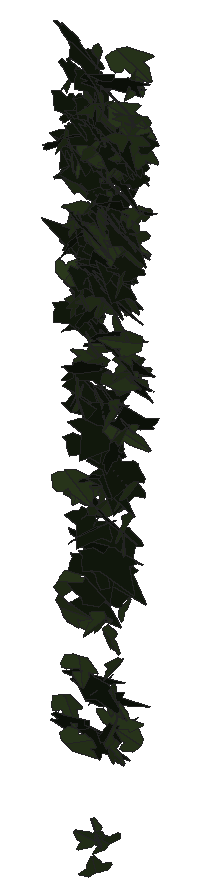
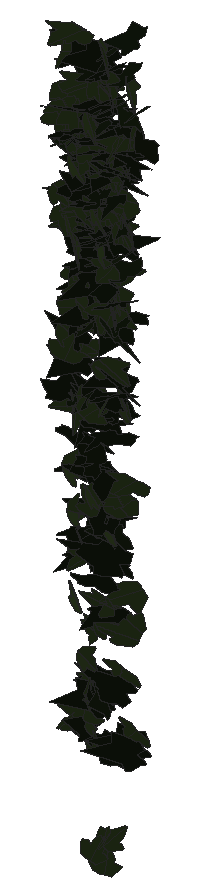
# SketchUp Ruby script. Lengths in millimetres.
U = 1.mm
M = Sketchup.active_model
def pt(a) = Geom::Point3d.new(a.map { |v| v * U })
def face(e, loops, mat)
  f = e.add_face(loops[0].map { |a| pt(a) })
  loops[1..].each { |l| e.add_face(l.map { |a| pt(a) }).erase! }
  f.material = f.back_material = mat if mat
  f
end
# faces: each face lists its corners as indices into pts; further lists are holes
def faces(e, pts, list, mat = nil) = list.each { |f| face(e, (f[0].is_a?(Array) ? f : [f]).map { |l| l.map { |i| pts[i] } }, mat) }
# xy, xz, yz: faces in a plane at the given z, y or x. An outline is a flat list of corners, or four numbers for a rectangle; further outlines are holes
def ring(l) = l.size == 4 ? [[l[0], l[1]], [l[2], l[1]], [l[2], l[3]], [l[0], l[3]]] : l.each_slice(2).to_a
def flat(e, list, mat, &to3) = list.each { |f| face(e, (f[0].is_a?(Array) ? f : [f]).map { |l| ring(l).map { |u, v| to3.(u, v) } }, mat) }
def xy(e, z, list, mat = nil) = flat(e, list, mat) { |x, y| [x, y, z] }
def xz(e, y, list, mat = nil) = flat(e, list, mat) { |x, z| [x, y, z] }
def yz(e, x, list, mat = nil) = flat(e, list, mat) { |y, z| [x, y, z] }
def lines(e, pts, list) = list.each { |a, b| e.add_line(pt(pts[a]), pt(pts[b])) }
# prism: a flat outline (further loops are holes) pulled along v
def prism(e, loops, v, mat = nil)
  f = face(e, loops, mat); d = Geom::Vector3d.new(v.map { |x| x * U })
  f.pushpull(f.normal.samedirection?(d) ? d.length : -d.length)
end
def box(e, o, s, mat = nil) = prism(e, [[o, [o[0] + s[0], o[1], o[2]], [o[0] + s[0], o[1] + s[1], o[2]], [o[0], o[1] + s[1], o[2]]]], [0, 0, s[2]], mat)
def at(x, y, z, deg = 0) = Geom::Transformation.translation(pt([x, y, z])) * Geom::Transformation.rotation(ORIGIN, Z_AXIS, deg.degrees)
def axes(o, x, y, z) = Geom::Transformation.new([*x, 0, *y, 0, *z, 0, *pt(o).to_a, 1])
def part(name) = M.definitions.add(name)
# library, detail: a bought-in or finely detailed component or shape, given as its bounding box
def library(name, o, s) = part(name).tap { |d| box(d.entities, o, s) }
def detail(e, o, s) = box(e.add_group.entities, o, s)
def put(e, d, t, mat = nil) = e.add_instance(d, t).tap { |i| i.material = mat if mat }
def group(e, t, mat = nil) = e.add_group.tap { |g| g.transformation = t; g.material = mat if mat }.entities
root = M.entities
M.materials.add("efeu1").color = [18, 25, 13]
M.materials.add("efeu2").color = [43, 57, 29]
c1 = part("ivyleaf_10")
p = [[0,12.8,-0.8],[-1.5,51.3,-10.9],[-4.9,51,-11.6],[-13.6,26.5,-7.3],[-13.2,15.9,-4.6],[-21.1,19.3,-7.2],
  [-29.5,16.3,-8.3],[-29.2,8.3,-6.2],[-19.7,-9.8,0.5],[-7.6,-13,4],[1,-12.2,5.8],[-0.4,51.1,-11.1],
  [-1.5,51.1,-10.9],[1,-12.4,5.9],[16.9,-12.4,3.5],[35.1,9.1,-5.1],[35,12.9,-6.1],[20.5,16.4,-4.9],
  [15.8,15,-3.8],[15.3,27.6,-7.1],[12.8,31.3,-7.8]]
faces(c1.entities,p,[[0,1,2,3,4,5,6,7,8,9,10],[11,12,0,13,14,15,16,17,18,19,20]],"efeu2")
c2 = part("ivyleaf_9")
p = [[39.1,54.8,31.7],[34.5,51.8,30.2],[-5.3,25.2,17.3],[-17.9,28.3,20.9],[-21.6,21.7,17],[-20.2,4.3,5.3],
  [-22.9,-0.3,2.5],[-17.1,-4,-0.6],[-2,-2.1,-1.2],[-0.7,-15.4,-10.1],[16.6,-22.3,-16.7],[21.1,-15.1,-12.5],
  [32.7,-10.7,-11],[46.1,-1.8,-6.6],[30.8,11.2,3.8]]
faces(c2.entities,p,[[0,1,2,3,4,5,6,7,8,9,10,11,12,13,14]],"efeu1")
put(root,c1,axes([2306.4,958.9,65.1],[-0.49268,-0.36082,-0.57278],[-0.62271,-0.47016,0.44405],[-1.12791,0.41718,0.00504]))
put(root,c1,axes([2262.1,935.2,1434.6],[-0.09896,-0.49853,-0.72888],[0.15767,0.72417,-0.50121],[1.67323,-0.09772,0.00412]))
put(root,c1,axes([2339.9,936.6,1299.7],[-0.34814,0.53797,0.53709],[-0.43479,0.48799,-0.56659],[-1.37991,-0.28948,0.04302]))
put(root,c2,axes([2364.3,933.3,858.2],[0.11458,-0.04516,-0.89711],[-1.05775,0.70448,-0.07276],[1.34302,0.55869,0.01923]))
put(root,c1,axes([2315,956.2,10],[-0.58701,-0.59557,-0.27554],[-0.24044,-0.24487,0.6707],[-1.22555,0.3333,0.00039]))
put(root,c1,axes([2391.6,960.3,1066.8],[-0.12621,-0.04578,-0.84309],[-1.31279,-0.48478,0.08058],[-0.92673,0.69296,0.00067]))
put(root,c2,axes([2326.7,937,1518.4],[0.06754,0.0188,-0.84588],[-1.42002,0.39992,-0.02242],[0.75932,0.74622,0.03332]))
put(root,c2,axes([2369.8,956.2,826.1],[-1.39765,-0.25317,-0.39205],[0.68805,0.15365,-0.7764],[0.56169,-0.81817,-0.02449]))
put(root,c1,axes([2370.8,960.3,1191],[0.433,-0.53815,0.4661],[0.34565,-0.42926,-0.58427],[1.31013,0.29111,0.0001]))
put(root,c2,axes([2307.6,962.7,686.4],[-0.82925,-0.62066,0.17912],[-0.18279,-0.15142,-0.75829],[1.21579,-0.4461,0.00817]))
put(root,c1,axes([2382.1,949.2,898.1],[0.07989,-0.81763,-0.16606],[-0.0415,0.16514,-0.81861],[1.58735,0.04547,-0.01304]))
put(root,c1,axes([2265.1,945.8,765],[1.24363,0.38111,0.45401],[0.69616,0.27249,-0.75519],[-0.88774,0.74757,0.04381]))
put(root,c1,axes([2339.9,961,258.8],[-0.14365,0.06886,-0.76785],[0.7937,-0.64524,-0.09886],[-1.23402,-0.42303,0.02579]))
put(root,c1,axes([2329.4,951.7,1511],[-0.57099,-0.84663,0.00578],[-0.0035,-0.00548,-0.89821],[1.61134,-0.30002,0.0001]))
put(root,c2,axes([2285.6,960.8,1596.7],[0.20531,-0.82442,0.12259],[0.05769,-0.11965,-0.83133],[1.58524,0.11113,0.01438]))
put(root,c1,axes([2247.9,956.1,496.2],[-0.64764,0.06535,0.7255],[1.33715,-0.18204,0.34593],[0.36614,0.78039,0.01994]))
put(root,c2,axes([2323.5,960.6,1292.1],[0.54514,-0.50862,0.53213],[0.58938,-0.43475,-0.58223],[1.27096,0.41976,0.04176]))
put(root,c2,axes([2312.2,955.2,610.5],[-0.91404,-0.30528,-0.63224],[1.06895,0.29255,-0.56791],[0.80174,-0.7381,0.0364]))
put(root,c1,axes([2342.6,961.6,352.1],[0.12018,-0.03133,0.7733],[1.18762,-0.45689,-0.06946],[0.8713,0.62708,-0.01198]))
put(root,c2,axes([2330.9,963.7,1539.4],[0.31518,-0.57207,0.58879],[0.5868,-0.51334,-0.58548],[1.44802,0.33254,0.1091]))
put(root,c1,axes([2360.7,960.5,1415.5],[-0.03448,-0.74129,0.37323],[0.13613,-0.37332,-0.738],[1.57367,0.01605,0.07202]))
put(root,c2,axes([2367.3,938.8,1578.5],[1.16505,0.56513,0.13133],[0.19397,0.08321,-0.83309],[-1.08706,0.62053,-0.0079]))
put(root,c2,axes([2348,951.5,786.5],[0.66856,-0.64102,-0.32987],[-0.30642,0.28793,-0.73096],[1.3374,0.38641,-0.00257]))
put(root,c1,axes([2324.6,940,1047.8],[-0.13988,-0.08981,-0.73061],[0.88419,0.56387,-0.11605],[1.08668,-0.47036,0.00038]))
put(root,c2,axes([2306.7,936,1092.5],[0.0999,0.44209,0.63564],[0.05692,0.63547,-0.44444],[-1.47248,0.05456,0.02594]))
put(root,c2,axes([2341.4,957.4,1181.5],[1.18471,-0.05553,0.53195],[-1.00217,0.07936,0.62447],[-0.17832,-0.81496,0.02456]))
put(root,c2,axes([2326.7,965.1,869.8],[-1.15879,-0.60672,0.12312],[-0.14494,-0.09798,-0.85941],[1.1693,-0.61342,0.01549]))
put(root,c1,axes([2281.5,956.7,1120.1],[0.17079,-0.89177,0.10539],[0.04625,-0.10347,-0.89616],[1.7084,0.09195,0.01373]))
put(root,c1,axes([2321.6,941.5,1038.5],[-0.23686,0.42105,-0.59435],[-0.50329,0.5357,0.43488],[1.29166,0.28594,0.06046]))
put(root,c1,axes([2388.8,951.2,1469.7],[-1.25192,-0.4557,-0.05778],[0.11272,0.01594,-0.79996],[0.86693,-0.66014,0.02057]))
put(root,c2,axes([2302.3,955.2,373.4],[-0.10895,-0.04436,-0.82621],[1.51762,0.21799,-0.06695],[0.42011,-0.79898,0.0276]))
put(root,c2,axes([2253,935.1,1424.6],[0.91317,0.7112,0.3862],[0.42487,0.31524,-0.85788],[-1.48048,0.52914,-0.00799]))
put(root,c1,axes([2275.1,956.3,403.8],[1.3541,-0.17134,0.27035],[0.50338,-0.05634,-0.7318],[0.34303,0.75903,0.0067]))
put(root,c2,axes([2322.7,956.3,1164],[0.57464,-0.69926,-0.17699],[-0.15447,0.15771,-0.76157],[1.36407,0.31243,-0.01169]))
put(root,c1,axes([2299.9,939.5,1136.5],[-0.23265,0.26561,0.72242],[-0.71916,0.61655,-0.29062],[-1.27621,-0.39585,0.03207]))
put(root,c2,axes([2336.6,953.1,634.5],[-0.43068,-0.50109,-0.65626],[0.68549,0.55241,-0.54598],[1.41407,-0.4204,0.0648]))
put(root,c1,axes([2335,952.3,1238.3],[1.01929,-0.23189,-0.50994],[-0.90114,0.18962,-0.58351],[0.56974,0.71478,-0.01063]))
put(root,c1,axes([2339.1,959,1331.4],[0.71851,-0.68155,0.1673],[0.15577,-0.14592,-0.77912],[1.32652,0.3863,0.00087]))
put(root,c2,axes([2244.5,960,1629.9],[0.95168,-0.69895,0.12172],[0.14261,-0.09605,-0.85939],[1.34272,0.5056,0.00501]))
put(root,c1,axes([2362.5,949.4,982.3],[-0.6751,-0.52179,0.45423],[0.45155,0.38775,0.6307],[-1.23679,0.42639,-0.01768]))
put(root,c1,axes([2313.4,952.9,1319.8],[0.13235,-0.75524,-0.18981],[0.06197,0.19322,-0.75687],[1.48077,0.05942,0.04864]))
put(root,c2,axes([2345.9,949.1,1435.6],[0.71762,-0.51834,-0.57077],[-0.56885,0.48742,-0.64009],[1.35264,0.47998,0.03362]))
put(root,c2,axes([2292.1,952.2,849.8],[-0.01846,-0.53903,-0.59916],[0.27403,0.5884,-0.53169],[1.5092,-0.11343,0.08921]))
put(root,c2,axes([2333.1,937.8,1060.8],[0.99668,0.38051,0.68488],[1.01112,0.43301,-0.6468],[-1.09596,0.74553,0.02611]))
put(root,c2,axes([2349.7,971.7,1166.7],[-0.57073,-0.57735,0.46408],[0.17755,-0.52612,-0.59425],[1.39857,-0.16882,0.26482]))
put(root,c2,axes([2280.7,954.4,1171],[0.70169,-0.62159,-0.33271],[-0.11659,0.34579,-0.71392],[1.33674,0.35645,0.11238]))
put(root,c2,axes([2315.5,965.3,1478.2],[0.40839,-0.77793,0.15754],[0.13852,-0.14323,-0.80637],[1.50426,0.22439,0.03148]))
put(root,c1,axes([2288.3,941.2,928.5],[-0.31168,0.22479,0.89507],[-1.21526,0.62872,-0.27473],[-1.26809,-0.65778,0.04329]))
put(root,c2,axes([2353,962.6,1457.9],[-0.34576,-0.01208,-0.80373],[1.52872,-0.03401,-0.18105],[-0.05808,-0.8233,0.01927]))
put(root,c2,axes([2311.5,944.6,1557.9],[1.04687,0.15062,0.6169],[1.10269,0.21502,-0.56911],[-0.49467,0.79806,0.0369]))
put(root,c1,axes([2262.5,942.1,1161.3],[0.61198,0.28852,-0.63424],[0.36914,0.63384,0.38668],[1.2737,-0.32233,0.19267]))
put(root,c2,axes([2270.5,957.6,1092.7],[-0.39574,-0.59761,-0.51311],[0.39568,0.47022,-0.63191],[1.44591,-0.29224,0.03249]))
put(root,c2,axes([2282.5,960.6,1239],[-0.42881,0.51676,-0.53556],[0.39076,-0.49469,-0.5637],[-1.36143,-0.30475,0.00689]))
put(root,c1,axes([2343.4,955.3,277.1],[0.61445,-0.76799,0.1296],[-0.09504,0.1196,0.83309],[-1.47925,-0.32669,0.00031]))
put(root,c1,axes([2301.7,961,1254.8],[-0.96415,0.31057,-0.50559],[0.66696,-0.37986,-0.58447],[-0.91128,-0.6066,0.10715]))
put(root,c1,axes([2325.3,957.5,1128.6],[-0.93487,-0.65682,0.02553],[-0.02903,-0.02047,-0.82018],[1.25066,-0.49144,0.00004]))
put(root,c2,axes([2313,960.2,1377.1],[1.1269,-0.54134,0.14898],[0.21056,-0.09978,-0.80227],[1.04764,0.60235,0.001]))
put(root,c1,axes([2346.3,974.4,915.6],[0.16756,-0.37842,0.85664],[0.47516,-0.81979,-0.38781],[1.71785,0.26367,0.02371]))
put(root,c2,axes([2326.2,969,1221.5],[-0.31714,-0.761,0.11539],[-0.00562,-0.11743,-0.77872],[1.46487,-0.1652,0.02199]))
put(root,c1,axes([2388.1,968,1027],[-0.28112,-0.68776,0.50868],[-0.17205,-0.50077,-0.70332],[1.61895,-0.17264,0.01359]))
put(root,c1,axes([2310.1,953,1406.5],[1.30656,0.11248,-0.49154],[0.9245,0.07522,0.69565],[0.25744,-0.84098,-0.00352]))
put(root,c2,axes([2253.9,960.4,1560.5],[0.8708,-0.69505,-0.09896],[-0.07819,0.09141,-0.83198],[1.33386,0.45912,0.01584]))
put(root,c2,axes([2296.8,961.3,1220.8],[-0.01863,0.0925,0.81453],[-1.55555,0.06158,-0.01681],[-0.12005,-0.81226,0.09148]))
put(root,c2,axes([2386.3,963.1,1220],[-1.36769,0.06407,0.43761],[-0.83493,0.00266,-0.72081],[-0.10678,-0.84138,0.03104]))
put(root,c2,axes([2301.6,963.8,1553.1],[0.05436,-0.81659,-0.19197],[-0.05508,0.19101,-0.81681],[1.59556,0.03441,-0.02166]))
put(root,c2,axes([2265.1,965.3,1270.2],[1.03589,-0.78141,0.18703],[0.18881,-0.15881,-0.95225],[1.51749,0.55318,-0.00919]))
put(root,c2,axes([2295.4,957.5,1453.8],[-0.08359,-0.58968,-0.56458],[0.38041,0.54042,-0.58],[1.50644,-0.16919,0.11513]))
put(root,c2,axes([2336.4,964.8,1055],[0.67121,-0.73903,0.03827],[0.03313,-0.0341,-0.81887],[1.40801,0.3531,0.00102]))
put(root,c1,axes([2305.9,974,1188.2],[0.12508,-0.35407,-0.79019],[0.23053,-0.78091,0.35999],[-1.63177,-0.13747,-0.00971]))
put(root,c1,axes([2311.3,954.4,1535.7],[1.19509,-0.42437,-0.34252],[-0.26517,0.38019,-0.72647],[1.00346,0.60587,0.21595]))
put(root,c1,axes([2262.8,962.9,905],[0.49836,-0.71309,-0.12686],[0.08368,-0.11899,0.75965],[-1.37592,-0.26552,0.00025]))
put(root,c2,axes([2364.6,961.2,1280.1],[0.40682,-0.72505,-0.31162],[-0.09139,0.3103,-0.75492],[1.49919,0.21566,0.03854]))
put(root,c1,axes([2310.1,974.6,489.3],[-0.0038,-0.30282,0.71041],[0.15738,-0.70641,-0.30089],[1.46131,0.07529,0.03425]))
put(root,c2,axes([2325,963.4,1228],[-0.60239,-0.60485,-0.43687],[0.35425,0.39554,-0.68248],[1.37512,-0.36686,-0.01556]))
put(root,c1,axes([2386.8,963.3,991.4],[-1.05882,-0.48954,0.26481],[-0.37666,-0.17595,-0.74105],[0.99003,-0.59049,0.00127]))
put(root,c2,axes([2242.5,968,1487.7],[0.31044,-0.82332,-0.03787],[-0.00209,0.03838,-0.8393],[1.5686,0.16299,0.00638]))
put(root,c1,axes([2290,966.2,1293.3],[-0.84575,-0.65768,0.26278],[-0.11124,-0.27511,-0.78738],[1.34331,-0.43686,0.10025]))
put(root,c1,axes([2272.3,967.3,1260.1],[-0.22311,-0.743,0.24242],[0.05368,-0.249,-0.74951],[1.48647,-0.10253,0.06345]))
put(root,c1,axes([2375.3,976.8,770.4],[0.29431,-0.56166,0.72735],[0.28271,-0.7126,-0.58185],[1.72598,0.21249,-0.02872]))
put(root,c1,axes([2328.7,971.3,470.7],[-0.28013,0.19766,-0.6896],[0.62361,-0.60772,-0.24413],[-1.21455,-0.35762,0.0337]))
put(root,c2,axes([2384.8,967.8,898.9],[1.04434,0.18542,0.54182],[-0.97085,-0.18278,0.57917],[0.49534,-0.74918,-0.0072]))
put(root,c2,axes([2344.8,969.3,1375.5],[0.68535,-0.7032,0.15678],[0.09391,-0.15079,-0.78967],[1.36798,0.36265,-0.02434]))
put(root,c1,axes([2287.3,969.4,659.7],[0.14512,-0.6073,-0.35431],[0.242,-0.3386,0.60773],[-1.31607,-0.12923,0.07268]))
put(root,c1,axes([2315.1,952.9,1426.2],[-0.50838,-0.54805,-0.55714],[0.55436,0.47655,-0.60842],[1.38021,-0.39327,0.03916]))
put(root,c1,axes([2347.9,960.5,1496.3],[-1.45122,-0.26645,0.11069],[-0.21436,-0.01306,-0.80736],[0.50556,-0.7704,-0.0246]))
put(root,c2,axes([2287.7,958.4,892.9],[-0.23123,0.00874,0.81576],[1.51789,-0.17226,0.12063],[0.32668,0.80657,0.01692]))
put(root,c2,axes([2306.4,964.7,1074.7],[0.98372,-0.65093,-0.05961],[-0.07383,0.04531,-0.83118],[1.24184,0.51833,-0.0022]))
put(root,c2,axes([2306.1,969.4,705.4],[0.88392,-0.54922,0.45596],[0.59049,-0.33458,-0.71905],[1.2235,0.55826,0.01763]))
put(root,c2,axes([2273.4,944.7,1477.6],[0.40889,0.45839,0.65824],[0.02212,0.67959,-0.47705],[-1.52643,0.13264,0.16941]))
put(root,c2,axes([2289.7,946.4,659.7],[-0.21321,0.64599,-0.46863],[-0.14726,0.46221,0.65563],[1.51174,0.13613,-0.00223]))
put(root,c2,axes([2332,956.5,547.9],[-1.5984,-0.05646,0.23177],[0.44037,0.01359,0.84174],[-0.11047,0.87114,0.00189]))
put(root,c1,axes([2364.6,965.7,1225.8],[-1.50236,-0.00174,0.28742],[0.54701,-0.01148,0.78931],[0.00436,0.84001,0.01138]))
put(root,c1,axes([2254.8,949.4,558.9],[-0.42445,-0.224,-0.88221],[1.08422,0.67406,-0.31516],[1.35106,-0.6113,-0.02425]))
put(root,c2,axes([2358.5,973.2,1016.9],[0.33075,-0.22307,0.73051],[0.76608,-0.60996,-0.28202],[1.23545,0.43795,-0.0207]))
put(root,c1,axes([2261.3,961.4,240],[0.90553,0.00884,-0.63596],[1.21014,0.01184,0.47587],[0.02813,-0.79415,0.00002]))
put(root,c2,axes([2237.8,959.7,275],[1.20585,-0.06482,0.47014],[0.88874,-0.05472,-0.63687],[0.1611,0.78706,-0.00556]))
put(root,c1,axes([2358.5,971.1,1400.7],[-0.665,-0.67022,0.29406],[-0.01538,-0.3223,-0.74419],[1.39286,-0.32355,0.13218]))
put(root,c2,axes([2287.5,970.8,1237.1],[0.35103,-0.76454,-0.04074],[-0.0017,0.04169,-0.78642],[1.45713,0.18423,0.0089]))
put(root,c1,axes([2255.7,963.7,1541.9],[0.25173,-0.8257,-0.16833],[0.00152,0.17052,-0.83579],[1.6038,0.12944,0.02721]))
put(root,c2,axes([2345.8,960.1,607.5],[0.17232,-0.55616,-0.63736],[0.11555,0.64362,-0.553],[1.60577,0.01337,0.10819]))
put(root,c1,axes([2341.7,975.5,1088.9],[0.08698,-0.17408,0.78669],[1.22665,-0.46496,-0.14033],[0.92023,0.63623,0.1127]))
put(root,c1,axes([2358.5,960.4,886],[0.65027,0.1764,0.68235],[1.18057,0.2847,-0.38421],[-0.63674,0.70801,-0.01551]))
put(root,c1,axes([2290.1,962.8,1242.4],[-0.84638,0.70787,-0.06223],[-0.07385,0.04911,0.83595],[1.3504,0.44635,0.00671]))
put(root,c2,axes([2296.6,968.3,1497.6],[0.25347,-0.79396,-0.27331],[0.04785,0.28038,-0.80223],[1.59738,0.11759,0.0674]))
put(root,c2,axes([2309.7,964.3,1362.9],[-1.50326,-0.33319,-0.19865],[-0.32068,-0.11122,0.8565],[-0.66499,0.80683,0.03603]))
put(root,c2,axes([2304,964.1,1144.2],[1.57695,-0.34182,0.18948],[0.32103,-0.08788,-0.89616],[0.67096,0.84541,-0.01654]))
put(root,c2,axes([2333.4,964.3,1271.9],[1.35679,-0.30211,0.154],[0.2612,-0.07078,-0.77419],[0.59015,0.7259,-0.01139]))
put(root,c2,axes([2317.4,965.3,1285.5],[0.8223,-0.62245,-0.24071],[-0.13331,0.24287,-0.75377],[1.26312,0.43085,0.07715]))
put(root,c2,axes([2268.2,963.4,368.6],[1.11645,0.32956,-0.39131],[0.61921,0.21914,0.67229],[0.75141,-0.67024,0.0274]))
put(root,c2,axes([2281.3,968.8,253.7],[0.75627,-0.07569,-0.68942],[1.28534,0.22307,0.36477],[0.30043,-0.76383,0.17485]))
put(root,c1,axes([2234.8,971.2,306.5],[1.1218,-0.1697,0.4472],[0.81644,-0.12637,-0.61337],[0.40268,0.72901,-0.00222]))
put(root,c2,axes([2322.8,974.7,1333.3],[-0.06764,-0.79116,-0.10623],[0.03478,0.1055,-0.79184],[1.51884,-0.03765,0.0134]))
put(root,c2,axes([2352,977.4,779.8],[-0.88177,-0.71241,-0.10635],[0.1071,0.09027,-0.84981],[1.36669,-0.46671,-0.00202]))
put(root,c1,axes([2345.1,976.2,417.7],[0.03916,-0.62016,0.37202],[0.00704,-0.37207,-0.62046],[1.37635,0.01955,-0.00741]))
put(root,c1,axes([2259.7,966.6,1273.7],[0.50171,-0.71139,-0.19754],[-0.12229,0.18685,-0.75865],[1.39982,0.27129,0.00452]))
put(root,c2,axes([2300.1,968.1,1459.5],[1.00589,-0.60117,-0.18155],[-0.16444,0.16542,-0.7993],[1.18382,0.53379,0.04324]))
put(root,c2,axes([2286.3,978.6,936.5],[-0.61902,-0.70375,0.01057],[0.00898,-0.01383,-0.77521],[1.33949,-0.32513,0.01008]))
put(root,c2,axes([2327.1,960.8,782.5],[0.48248,0.74846,-0.2114],[-0.13017,-0.20003,-0.79022],[-1.47446,0.26257,0.00059]))
put(root,c1,axes([2270.8,971.3,742.2],[0.82676,0.50582,-0.23347],[-0.31974,-0.16333,-0.66646],[-1.01091,0.46534,0.01985]))
put(root,c2,axes([2310.7,979.6,801.2],[0.84523,-0.13885,-0.6961],[1.25317,-0.22608,0.46519],[-0.50454,-0.79416,-0.01072]))
put(root,c2,axes([2262.2,974.8,1212],[0.36932,-0.73731,-0.05239],[-0.0219,0.05115,-0.76241],[1.40661,0.19438,0.00188]))
put(root,c1,axes([2382.5,982.9,1571.1],[0.07826,0.43246,-0.78849],[-0.23633,-0.77903,-0.43374],[-1.69516,0.12857,0.02407]))
put(root,c1,axes([2267.1,967.1,719.7],[-0.91719,-0.35196,0.41518],[0.6288,0.25151,0.59672],[-0.8232,0.58426,-0.00677]))
put(root,c2,axes([2334.2,971.2,1176.6],[-0.20982,-0.68489,-0.45434],[0.16853,0.44584,-0.69357],[1.55511,-0.14072,0.01386]))
put(root,c2,axes([2335.4,980.8,1467.3],[-0.44173,-0.07874,0.763],[-1.36562,-0.25948,-0.24505],[0.516,-0.75413,0.00465]))
put(root,c2,axes([2277.5,963.2,1071.6],[1.45088,-0.0328,-0.37748],[-0.71328,0.05955,-0.76205],[0.10614,0.84859,0.03888]))
put(root,c1,axes([2315.7,969.4,707.4],[-0.50543,-0.77695,0.23113],[0.2276,0.203,0.81981],[-1.52585,0.28764,0.04573]))
put(root,c1,axes([2320.2,974.2,1284.2],[0.05554,-0.79936,0.0857],[0.01325,-0.0855,-0.79989],[1.53001,0.02976,0.00381]))
put(root,c2,axes([2305.8,982.4,1313.3],[0.53066,-0.66473,0.43253],[0.27978,-0.40722,-0.7206],[1.4832,0.31464,-0.01883]))
put(root,c1,axes([2298.8,971.7,85.9],[-0.31483,0.66989,-0.17543],[0.08139,-0.17014,-0.69001],[-1.31541,-0.17086,-0.0007]))
put(root,c1,axes([2357.3,959.7,1508.8],[0.59548,0.39375,0.66475],[0.59351,0.59181,-0.49733],[-1.34534,0.43537,0.07483]))
put(root,c2,axes([2325.6,959.5,1303.3],[0.83561,0.11727,0.70979],[1.26221,0.25625,-0.45257],[-0.53057,0.7943,0.04121]))
put(root,c1,axes([2382.9,973,1495.4],[-0.93105,-0.66717,0.05283],[0.01668,-0.07182,-0.82582],[1.27362,-0.48678,0.04944]))
put(root,c1,axes([2380.6,978.5,273.4],[-0.02635,0.59627,0.47066],[-0.03985,-0.47086,0.5959],[1.4452,-0.00211,0.02501]))
put(root,c2,axes([2270,960,979],[1.13834,0.33004,0.3442],[0.57795,0.16211,-0.68312],[-0.69977,0.67078,-0.00427]))
put(root,c2,axes([2340.9,957.3,273.6],[0.01261,0.03793,0.80643],[1.04802,0.58952,-0.03225],[-1.12359,0.5503,-0.02103]))
put(root,c1,axes([2334.8,963.3,1132.8],[-0.64965,-0.27715,-0.64569],[0.99194,0.38158,-0.43931],[0.8969,-0.62276,0.01818]))
put(root,c1,axes([2329.6,984.9,351.5],[0.27989,-0.39968,0.69972],[0.77946,-0.57549,-0.4148],[1.3208,0.42432,0.09651]))
put(root,c1,axes([2306.8,971.4,1596.1],[0.59311,-0.76022,-0.18841],[-0.01371,0.19998,-0.81884],[1.49056,0.30434,0.06744]))
put(root,c2,axes([2343.2,981.5,1286.8],[-1.17196,-0.06983,0.43979],[-0.80136,-0.15294,-0.61384],[0.27581,-0.74109,0.08524]))
put(root,c1,axes([2358.6,988.5,696.5],[0.3198,-0.43379,0.74037],[0.44665,-0.70244,-0.46483],[1.57086,0.28804,-0.01856]))
put(root,c2,axes([2241.7,986.7,1192.2],[0.0798,-0.62521,0.47513],[0.36084,-0.45367,-0.6137],[1.45029,0.14728,0.12655]))
put(root,c1,axes([2268.7,980.6,1127],[-0.38995,0.5131,-0.49031],[0.16503,-0.48841,-0.54735],[-1.34058,-0.20937,0.07524]))
put(root,c1,axes([2294.5,980.1,995.5],[-0.75276,-0.42422,0.48369],[-0.60217,-0.36611,-0.57983],[1.06615,-0.50631,0.01401]))
put(root,c1,axes([2359.3,966.6,1250.8],[-0.35512,-0.42334,-0.62517],[1.08916,0.34075,-0.40155],[0.9373,-0.55636,0.22975]))
put(root,c2,axes([2336.7,963.1,1304.6],[-0.2716,-0.17651,0.84402],[1.37977,0.4386,0.2143],[-0.88848,0.73509,0.0748]))
put(root,c1,axes([2243.6,980,1328.1],[-0.57209,0.19641,-0.75857],[1.1472,-0.46117,-0.35826],[-0.95288,-0.67314,0.02411]))
put(root,c2,axes([2275.7,966.5,1334.6],[1.09265,-0.19969,-0.53388],[-0.88868,0.26982,-0.60305],[0.62217,0.73609,0.07622]))
put(root,c1,axes([2365.7,970.2,1140.8],[-1.1792,0.35525,0.16784],[-0.30649,0.05627,-0.71356],[-0.68207,-0.63945,0.03046]))
put(root,c1,axes([2330.5,972.4,1418.6],[1.25793,0.3724,0.21897],[0.31791,0.1488,-0.75726],[-0.75824,0.6802,0.04577]))
put(root,c1,axes([2298.9,977.7,927.6],[-0.50836,0.68467,-0.33979],[0.23525,-0.31651,-0.73493],[-1.43556,-0.29432,-0.00011]))
put(root,c1,axes([2316.9,987.2,50.3],[-0.4587,-0.46735,-0.58776],[-0.39854,-0.55097,0.52397],[-1.37245,0.31619,0.04429]))
put(root,c2,axes([2281.1,988.4,1119.6],[-0.75333,-0.61012,0.23934],[-0.14023,-0.2364,-0.7245],[1.23943,-0.39758,0.0635]))
put(root,c1,axes([2346.4,987.2,663.4],[0.26359,-0.21962,0.72972],[0.89909,-0.55722,-0.25737],[1.13804,0.4911,0.03431]))
put(root,c2,axes([2312.9,971.7,1404.9],[-1.20859,-0.42973,0.35723],[0.61619,0.15782,0.76539],[-0.86687,0.71132,0.046]))
put(root,c1,axes([2375.8,983.7,990.2],[-0.96361,-0.48638,-0.37022],[-0.44849,-0.28825,0.70097],[-1.0734,0.55707,0.03947]))
put(root,c1,axes([2251.8,969.5,484.1],[-0.26898,-0.09611,0.7972],[1.29451,0.41588,0.17072],[-0.81222,0.69465,0.00808]))
put(root,c2,axes([2299.4,977.6,915.4],[-0.36956,0.04581,0.74962],[1.14356,-0.45503,0.18345],[0.8575,0.62657,0.07841]))
put(root,c2,axes([2267.5,983.5,1407.6],[-1.44569,-0.27683,-0.11932],[0.20607,0.05132,-0.8084],[0.53543,-0.76721,-0.01102]))
put(root,c2,axes([2362.7,968.7,984.4],[1.43624,0.09488,-0.06699],[-0.12873,0.00101,-0.76053],[-0.1797,0.75761,0.0094]))
put(root,c1,axes([2285.1,975,1367.3],[0.6497,0.71991,-0.0217],[-0.01368,-0.02061,-0.79674],[-1.37069,0.34144,-0.00234]))
put(root,c2,axes([2313.1,982.3,1370],[-1.5606,-0.00074,0.27979],[-0.53249,0.00771,-0.81995],[-0.0034,-0.86637,-0.00754]))
put(root,c1,axes([2374,975.5,1247],[0.0717,-0.74397,-0.14396],[-0.00685,0.14396,-0.74491],[1.44217,0.03767,0.00362]))
put(root,c1,axes([2386.8,976.6,1435.9],[-1.52647,-0.11083,0.10074],[-0.15703,-0.13107,-0.80109],[0.23789,-0.79766,0.11763]))
put(root,c2,axes([2269.4,984.8,1412],[-0.6023,-0.71563,-0.13253],[0.09717,0.12233,-0.78248],[1.38173,-0.32055,-0.00274]))
put(root,c1,axes([2358,975.9,1449.7],[-1.24526,-0.46309,0.03838],[-0.06765,-0.0162,-0.80156],[0.88178,-0.65522,-0.0073]))
put(root,c1,axes([2268.8,967.4,1428.3],[-0.09262,-0.59501,-0.55283],[0.46112,0.51797,-0.57882],[1.47538,-0.19924,0.1462]))
put(root,c1,axes([2338,966.9,610.9],[0.42704,0.59132,0.48602],[0.35807,0.44833,-0.63232],[-1.41208,0.29251,-0.01336]))
put(root,c2,axes([2292.5,981.6,684.2],[0.48336,0.44224,0.57746],[-0.75957,-0.42661,0.50225],[1.15729,-0.46472,0.08846]))
put(root,c2,axes([2358.6,981.6,899.7],[0.27949,-0.82199,0.35173],[-0.07664,0.35,0.83477],[-1.6999,-0.15093,0.0202]))
put(root,c2,axes([2340.9,986.2,1416.8],[-1.22764,-0.46675,-0.16169],[0.29433,0.06176,-0.79521],[0.89286,-0.66212,0.03981]))
put(root,c2,axes([2394.4,988.3,1460.6],[-1.32784,-0.06374,0.38908],[-0.63918,-0.31818,-0.65436],[0.39306,-0.73274,0.25029]))
put(root,c2,axes([2288.5,970.2,522.4],[0.03035,-0.34438,-0.6838],[0.05566,0.68372,-0.34366],[1.45608,-0.01896,0.02739]))
put(root,c1,axes([2345.6,974.9,300.6],[1.45858,0.1115,0.03958],[-0.07455,-0.00567,0.77445],[0.21247,-0.76739,0.00002]))
put(root,c2,axes([2340.2,983.5,667.5],[-0.31473,-0.7849,-0.26819],[0.06112,0.26721,-0.80182],[1.57744,-0.16695,-0.02244]))
put(root,c1,axes([2322.7,990,898.2],[-0.60997,-0.23206,-0.65993],[-0.77198,-0.52976,0.38328],[-1.08471,0.50752,0.09832]))
put(root,c2,axes([2280,978.1,1495.3],[0.59993,-0.69824,-0.32345],[0.00027,0.34959,-0.75452],[1.46454,0.28596,0.13264]))
put(root,c2,axes([2257.9,989.7,1084.9],[0.37559,-0.60262,0.41738],[0.24986,-0.3962,-0.63411],[1.37257,0.23702,0.00122]))
put(root,c2,axes([2313.4,965.1,1144.8],[0.21905,-0.15435,-0.89731],[-0.05504,0.90337,-0.1591],[1.73196,0.04823,0.10843]))
put(root,c1,axes([2355.7,978.8,1287.8],[-1.30854,-0.05511,0.38302],[-0.70501,-0.1321,-0.68395],[0.21298,-0.77587,0.08924]))
put(root,c1,axes([2290.2,984.9,538.6],[-0.22907,0.03541,-0.73913],[1.14482,-0.43146,-0.11862],[-0.82024,-0.61209,0.04086]))
put(root,c2,axes([2302.6,981.4,980.5],[-1.46291,0.26052,-0.00953],[0.01716,-0.00307,-0.81161],[-0.49586,-0.76871,0.00001]))
put(root,c2,axes([2392.5,981,1389.3],[-1.25987,0.42777,-0.04278],[-0.08741,-0.14846,-0.77388],[-0.81352,-0.64653,0.14939]))
put(root,c1,axes([2267,971.8,1429.9],[0.69111,0.65044,0.29531],[0.06759,0.31443,-0.73622],[-1.35786,0.34671,0.11366]))
put(root,c2,axes([2312.8,966.9,341.2],[1.04443,0.22463,0.5522],[0.96309,0.22122,-0.59289],[-0.59975,0.74642,0.00954]))
put(root,c1,axes([2324.9,986.3,1380.8],[-0.42188,-0.71925,0.27722],[0.16002,-0.3093,-0.73524],[1.45829,-0.17414,0.16088]))
put(root,c1,axes([2297.8,974.9,1376.5],[-1.14711,0.50627,0.13738],[-0.24415,0.06065,-0.78634],[-0.96807,-0.6152,0.03553]))
put(root,c1,axes([2256.1,975,1376.1],[-0.04799,0.77112,0.12282],[-0.13701,0.12006,-0.7686],[-1.47976,-0.03613,0.06718]))
put(root,c2,axes([2237.3,973.9,265.4],[1.17989,-0.01156,0.4639],[0.88308,0.00372,-0.61998],[0.01337,0.77429,0.00991]))
put(root,c1,axes([2282.8,977.5,1380.4],[-1.37322,0.24589,0.17205],[-0.3651,-0.03337,-0.75681],[-0.43923,-0.74101,0.09117]))
put(root,c1,axes([2380.4,982.7,1472.1],[0.74519,0.66223,-0.25685],[-0.43278,-0.16099,-0.76171],[-1.28069,0.43973,0.10795]))
put(root,c1,axes([2284,977.8,1100.9],[-1.58642,-0.12212,-0.11742],[0.22114,0.01695,-0.84245],[0.23464,-0.84161,0.00007]))
put(root,c2,axes([2290.6,980.6,1078],[-1.11438,0.59707,-0.21516],[0.26754,-0.16346,-0.83615],[-1.17787,-0.60202,0.01364]))
put(root,c1,axes([2360.8,973.8,1611],[0.99684,0.47337,0.55455],[0.76589,0.3817,-0.70591],[-1.15714,0.66043,0.0105]))
put(root,c2,axes([2269.1,982.7,624.9],[0.86393,-0.25146,0.74257],[1.27331,-0.32306,-0.51839],[0.77784,0.80815,0.02383]))
put(root,c1,axes([2363.6,975.7,1205.3],[0.2987,-0.66236,-0.39426],[-0.14212,0.3874,-0.68055],[1.46013,0.17321,0.01441]))
put(root,c1,axes([2346.7,988.8,518.2],[0.24691,-0.60881,-0.37491],[0.27215,-0.35124,0.61985],[-1.33327,-0.18444,0.0571]))
put(root,c2,axes([2286.1,990.9,1369.7],[-1.44907,-0.19307,0.15907],[-0.25852,-0.10885,-0.78229],[0.3998,-0.77017,0.07069]))
put(root,c2,axes([2289.1,973.6,1384.3],[1.3177,0.31292,-0.17973],[-0.30242,-0.08477,-0.7597],[-0.61663,0.71027,-0.01149]))
put(root,c2,axes([2360.2,991.9,1426.7],[-0.65561,-0.72407,-0.02238],[0.01962,0.01988,-0.80183],[1.37856,-0.34463,0.00077]))
put(root,c2,axes([2256.8,991.3,1377.5],[0.06881,-0.7984,0.06051],[0.0169,-0.06017,-0.7992],[1.52378,0.03672,0.00613]))
put(root,c1,axes([2379.2,981.1,1262.4],[-0.74343,-0.68014,-0.06591],[0.0514,0.06049,-0.7843],[1.29948,-0.3915,-0.00669]))
put(root,c2,axes([2349.4,984.8,1424.3],[0.53889,-0.72603,-0.20516],[-0.05718,0.2081,-0.77793],[1.43474,0.28099,0.04605]))
put(root,c1,axes([2319.8,986.7,1402.3],[-0.79959,-0.63714,0.21631],[-0.11852,-0.2171,-0.76042],[1.27509,-0.41972,0.06496]))
put(root,c1,axes([2326,983.7,1460.5],[-0.05523,-0.81791,-0.02892],[0.00092,0.02892,-0.81843],[1.55762,-0.02902,-0.00054]))
put(root,c1,axes([2356.7,976.1,886.1],[0.00603,-0.65593,-0.41451],[0.1507,0.41262,-0.65234],[1.46903,-0.03964,0.06862]))
put(root,c2,axes([2313.6,982.4,1399.6],[0.22166,-0.66884,-0.43019],[0.19326,0.44373,-0.6624],[1.50111,0.04164,0.1488]))
put(root,c2,axes([2304.1,966.7,340.9],[0.2989,0.21496,0.73889],[0.46505,0.70116,-0.25592],[-1.38876,0.28106,0.07333]))
put(root,c1,axes([2276.9,980.5,1106.9],[0.34468,-0.70138,-0.23666],[0.01455,0.2454,-0.72143],[1.40873,0.16907,0.06536]))
put(root,c1,axes([2385.7,991.7,1307.6],[-0.38884,-0.64905,0.38443],[-0.0635,-0.39011,-0.67638],[1.43428,-0.19323,0.07427]))
put(root,c1,axes([2283,983.5,1187],[-1.15177,0.36773,-0.23142],[0.3317,-0.15802,-0.70687],[-0.75748,-0.62835,0.04233]))
put(root,c1,axes([2355.6,989,1370.7],[0.08025,-0.76807,0.17268],[-0.00146,-0.17297,-0.76916],[1.49827,0.04097,-0.01]))
put(root,c1,axes([2316.1,991.1,748.5],[0.13653,-0.71504,0.26849],[0.11107,-0.26375,-0.71801],[1.44939,0.08757,0.02973]))
